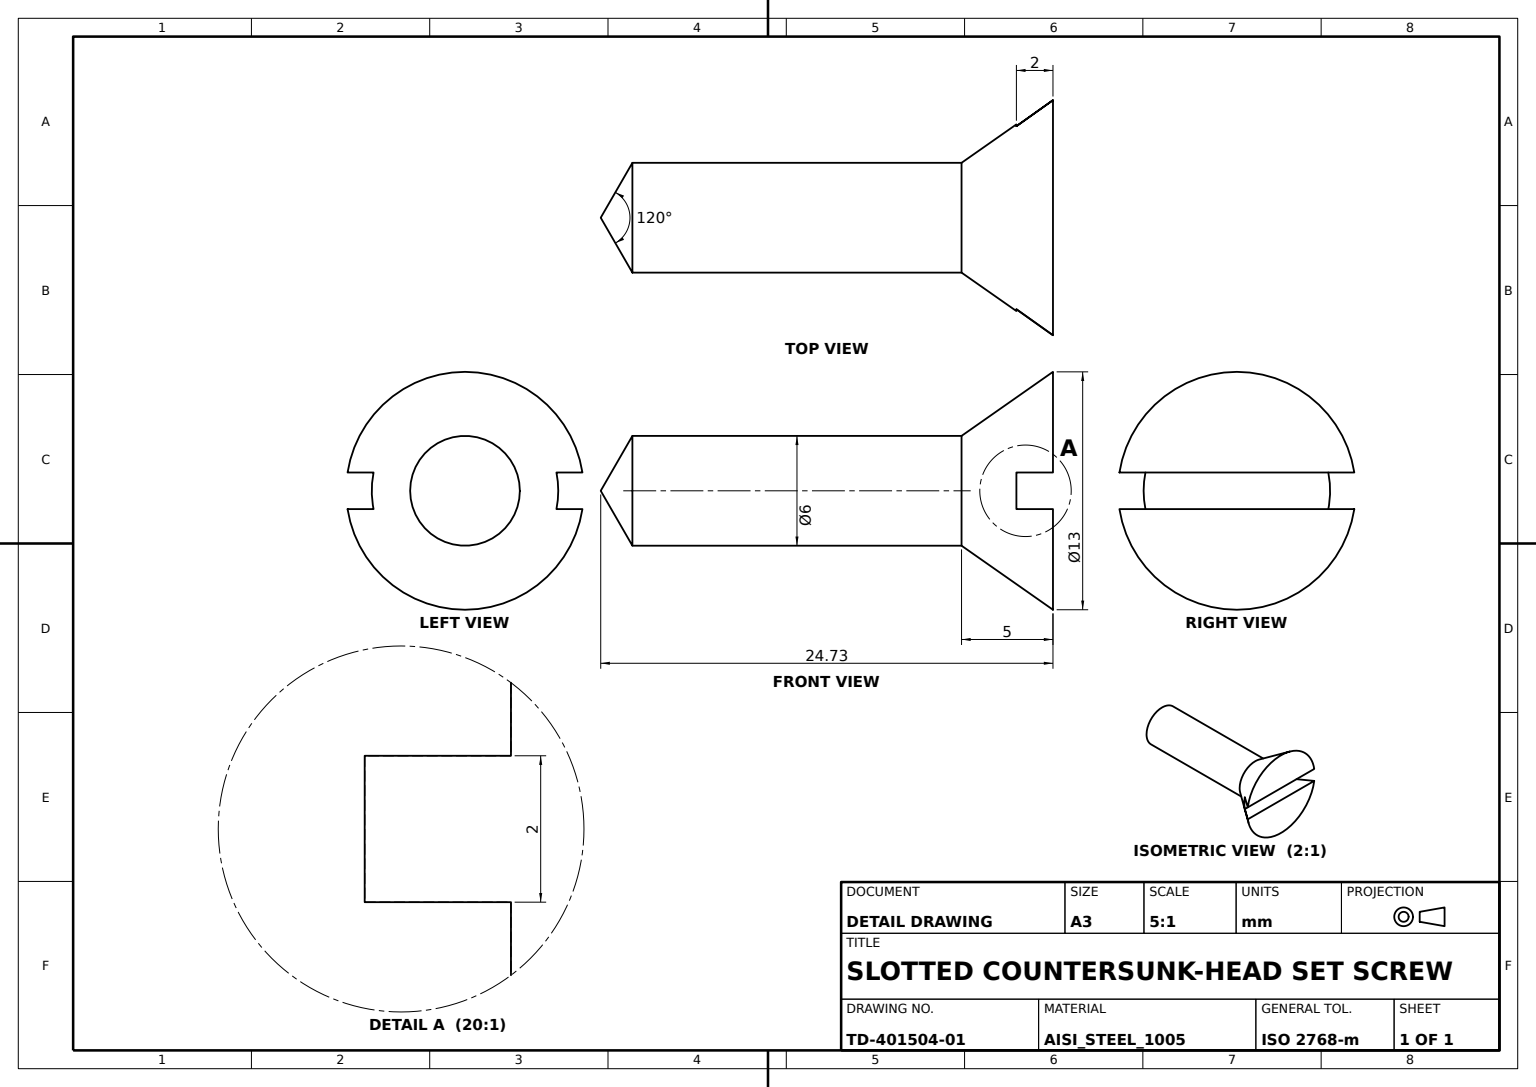
ISO-10303-21;
HEADER;
FILE_DESCRIPTION((''),'2;1');
FILE_NAME('','',(''),(''),'','','');
FILE_SCHEMA(('AUTOMOTIVE_DESIGN'));
ENDSEC;
DATA;
#1=APPLICATION_CONTEXT('');
#2=PRODUCT_CONTEXT('',#1,'mechanical');
#3=PRODUCT('','','',(#2));
#4=PRODUCT_DEFINITION_FORMATION('','',#3);
#5=PRODUCT_DEFINITION_CONTEXT('',#1,'design');
#6=PRODUCT_DEFINITION('','',#4,#5);
#7=PRODUCT_DEFINITION_SHAPE('','',#6);
#8=(LENGTH_UNIT()NAMED_UNIT(*)SI_UNIT(.MILLI.,.METRE.));
#9=(NAMED_UNIT(*)PLANE_ANGLE_UNIT()SI_UNIT($,.RADIAN.));
#10=(NAMED_UNIT(*)SI_UNIT($,.STERADIAN.)SOLID_ANGLE_UNIT());
#11=UNCERTAINTY_MEASURE_WITH_UNIT(LENGTH_MEASURE(0.005),#8,'distance_accuracy_value','');
#12=(GEOMETRIC_REPRESENTATION_CONTEXT(3)GLOBAL_UNCERTAINTY_ASSIGNED_CONTEXT((#11))GLOBAL_UNIT_ASSIGNED_CONTEXT((#8,#9,#10))REPRESENTATION_CONTEXT('',''));
#13=CARTESIAN_POINT('',(-13.646654,0.,-3.));
#14=VERTEX_POINT('',#13);
#15=CARTESIAN_POINT('',(-13.646654,0.,0.));
#16=DIRECTION('',(1.,0.,0.));
#17=DIRECTION('',(0.,0.,-1.));
#18=AXIS2_PLACEMENT_3D('',#15,#16,#17);
#19=CIRCLE('',#18,3.);
#20=EDGE_CURVE('',#14,#14,#19,.T.);
#21=ORIENTED_EDGE('',*,*,#20,.T.);
#22=EDGE_LOOP('',(#21));
#23=FACE_BOUND('',#22,.T.);
#24=CARTESIAN_POINT('',(4.353346,0.,-3.));
#25=VERTEX_POINT('',#24);
#26=CARTESIAN_POINT('',(4.353346,0.,0.));
#27=AXIS2_PLACEMENT_3D('',#26,#16,#17);
#28=CIRCLE('',#27,3.);
#29=EDGE_CURVE('',#25,#25,#28,.T.);
#30=ORIENTED_EDGE('',*,*,#29,.F.);
#31=EDGE_LOOP('',(#30));
#32=FACE_BOUND('',#31,.T.);
#33=CARTESIAN_POINT('',(0.,0.,0.));
#34=AXIS2_PLACEMENT_3D('',#33,#16,#17);
#35=CYLINDRICAL_SURFACE('',#34,3.);
#36=ADVANCED_FACE('',(#23,#32),#35,.T.);
#37=ORIENTED_EDGE('',*,*,#20,.F.);
#38=EDGE_LOOP('',(#37));
#39=FACE_BOUND('',#38,.T.);
#40=CARTESIAN_POINT('',(-16.646654,-1.,-5.001));
#41=VERTEX_POINT('',#40);
#42=CARTESIAN_POINT('',(-16.646654,1.,-5.001));
#43=VERTEX_POINT('',#42);
#44=CARTESIAN_POINT('',(-16.646654,0.,0.));
#45=DIRECTION('',(-1.,0.,0.));
#46=DIRECTION('',(0.,0.,1.));
#47=AXIS2_PLACEMENT_3D('',#44,#45,#46);
#48=CIRCLE('',#47,5.1);
#49=EDGE_CURVE('',#41,#43,#48,.F.);
#50=ORIENTED_EDGE('',*,*,#49,.T.);
#51=CARTESIAN_POINT('',(-18.646654,1.,-6.422616));
#52=VERTEX_POINT('',#51);
#53=CARTESIAN_POINT('',(-17.312348,1.,-5.47621));
#54=CARTESIAN_POINT('',(-17.979237,1.,-5.949795));
#55=B_SPLINE_CURVE_WITH_KNOTS('',3,(#42,#53,#54,#51),.UNSPECIFIED.,.F.,.F.,(4,4),(0.027715114,0.030169137),.UNSPECIFIED.);
#56=EDGE_CURVE('',#43,#52,#55,.T.);
#57=ORIENTED_EDGE('',*,*,#56,.T.);
#58=CARTESIAN_POINT('',(-18.646654,1.,6.422616));
#59=VERTEX_POINT('',#58);
#60=CARTESIAN_POINT('',(-18.646654,0.,0.));
#61=AXIS2_PLACEMENT_3D('',#60,#16,#17);
#62=CIRCLE('',#61,6.5);
#63=EDGE_CURVE('',#52,#59,#62,.T.);
#64=ORIENTED_EDGE('',*,*,#63,.T.);
#65=CARTESIAN_POINT('',(-16.646654,1.,5.001));
#66=VERTEX_POINT('',#65);
#67=CARTESIAN_POINT('',(-17.979241,1.,5.949798));
#68=CARTESIAN_POINT('',(-17.312364,1.,5.476222));
#69=B_SPLINE_CURVE_WITH_KNOTS('',3,(#58,#67,#68,#65),.UNSPECIFIED.,.F.,.F.,(4,4),(0.009653863,0.012107633),.UNSPECIFIED.);
#70=EDGE_CURVE('',#59,#66,#69,.T.);
#71=ORIENTED_EDGE('',*,*,#70,.T.);
#72=CARTESIAN_POINT('',(-16.646654,-1.,5.001));
#73=VERTEX_POINT('',#72);
#74=EDGE_CURVE('',#66,#73,#48,.F.);
#75=ORIENTED_EDGE('',*,*,#74,.T.);
#76=CARTESIAN_POINT('',(-18.646654,-1.,6.422616));
#77=VERTEX_POINT('',#76);
#78=CARTESIAN_POINT('',(-17.312348,-1.,5.47621));
#79=CARTESIAN_POINT('',(-17.979237,-1.,5.949795));
#80=B_SPLINE_CURVE_WITH_KNOTS('',3,(#72,#78,#79,#76),.UNSPECIFIED.,.F.,.F.,(4,4),(0.027715114,0.030169137),.UNSPECIFIED.);
#81=EDGE_CURVE('',#73,#77,#80,.T.);
#82=ORIENTED_EDGE('',*,*,#81,.T.);
#83=CARTESIAN_POINT('',(-18.646654,-1.,-6.422616));
#84=VERTEX_POINT('',#83);
#85=EDGE_CURVE('',#77,#84,#62,.T.);
#86=ORIENTED_EDGE('',*,*,#85,.T.);
#87=CARTESIAN_POINT('',(-17.979241,-1.,-5.949798));
#88=CARTESIAN_POINT('',(-17.312364,-1.,-5.476222));
#89=B_SPLINE_CURVE_WITH_KNOTS('',3,(#83,#87,#88,#40),.UNSPECIFIED.,.F.,.F.,(4,4),(0.009653863,0.012107633),.UNSPECIFIED.);
#90=EDGE_CURVE('',#84,#41,#89,.T.);
#91=ORIENTED_EDGE('',*,*,#90,.T.);
#92=EDGE_LOOP('',(#50,#57,#64,#71,#75,#82,#86,#91));
#93=FACE_BOUND('',#92,.T.);
#94=AXIS2_PLACEMENT_3D('',#15,#45,#46);
#95=CONICAL_SURFACE('',#94,3.,0.610725964);
#96=ADVANCED_FACE('',(#39,#93),#95,.T.);
#97=CARTESIAN_POINT('',(-16.646654,1.,7.));
#98=VECTOR('',#17,1000.);
#99=LINE('',#97,#98);
#100=EDGE_CURVE('',#43,#66,#99,.F.);
#101=ORIENTED_EDGE('',*,*,#100,.F.);
#102=ORIENTED_EDGE('',*,*,#49,.F.);
#103=CARTESIAN_POINT('',(-16.646654,-1.,7.));
#104=LINE('',#103,#98);
#105=EDGE_CURVE('',#41,#73,#104,.F.);
#106=ORIENTED_EDGE('',*,*,#105,.T.);
#107=ORIENTED_EDGE('',*,*,#74,.F.);
#108=EDGE_LOOP('',(#101,#102,#106,#107));
#109=FACE_BOUND('',#108,.T.);
#110=AXIS2_PLACEMENT_3D('',#103,#45,#46);
#111=PLANE('',#110);
#112=ADVANCED_FACE('',(#109),#111,.T.);
#113=ORIENTED_EDGE('',*,*,#85,.F.);
#114=CARTESIAN_POINT('',(-18.646654,-1.,7.));
#115=LINE('',#114,#98);
#116=EDGE_CURVE('',#77,#84,#115,.T.);
#117=ORIENTED_EDGE('',*,*,#116,.T.);
#118=EDGE_LOOP('',(#113,#117));
#119=FACE_BOUND('',#118,.T.);
#120=CARTESIAN_POINT('',(-18.646654,6.5,0.));
#121=AXIS2_PLACEMENT_3D('',#120,#45,#46);
#122=PLANE('',#121);
#123=ADVANCED_FACE('',(#119),#122,.T.);
#124=ORIENTED_EDGE('',*,*,#63,.F.);
#125=CARTESIAN_POINT('',(-18.646654,1.,7.));
#126=LINE('',#125,#98);
#127=EDGE_CURVE('',#59,#52,#126,.T.);
#128=ORIENTED_EDGE('',*,*,#127,.F.);
#129=EDGE_LOOP('',(#124,#128));
#130=FACE_BOUND('',#129,.T.);
#131=ADVANCED_FACE('',(#130),#122,.T.);
#132=CARTESIAN_POINT('',(6.085396,0.,0.));
#133=VERTEX_POINT('',#132);
#134=VERTEX_LOOP('',#133);
#135=FACE_BOUND('',#134,.T.);
#136=ORIENTED_EDGE('',*,*,#29,.T.);
#137=EDGE_LOOP('',(#136));
#138=FACE_BOUND('',#137,.T.);
#139=AXIS2_PLACEMENT_3D('',#132,#45,#46);
#140=CONICAL_SURFACE('',#139,0.,1.047197551);
#141=ADVANCED_FACE('',(#135,#138),#140,.T.);
#142=ORIENTED_EDGE('',*,*,#70,.F.);
#143=ORIENTED_EDGE('',*,*,#127,.T.);
#144=ORIENTED_EDGE('',*,*,#56,.F.);
#145=ORIENTED_EDGE('',*,*,#100,.T.);
#146=EDGE_LOOP('',(#142,#143,#144,#145));
#147=FACE_BOUND('',#146,.T.);
#148=DIRECTION('',(0.,-1.,0.));
#149=AXIS2_PLACEMENT_3D('',#97,#148,#17);
#150=PLANE('',#149);
#151=ADVANCED_FACE('',(#147),#150,.T.);
#152=ORIENTED_EDGE('',*,*,#81,.F.);
#153=ORIENTED_EDGE('',*,*,#105,.F.);
#154=ORIENTED_EDGE('',*,*,#90,.F.);
#155=ORIENTED_EDGE('',*,*,#116,.F.);
#156=EDGE_LOOP('',(#152,#153,#154,#155));
#157=FACE_BOUND('',#156,.T.);
#158=DIRECTION('',(0.,1.,0.));
#159=AXIS2_PLACEMENT_3D('',#114,#158,#46);
#160=PLANE('',#159);
#161=ADVANCED_FACE('',(#157),#160,.T.);
#162=CLOSED_SHELL('',(#36,#96,#112,#123,#131,#141,#151,#161));
#163=MANIFOLD_SOLID_BREP('',#162);
#164=ADVANCED_BREP_SHAPE_REPRESENTATION('',(#163),#12);
#165=SHAPE_DEFINITION_REPRESENTATION(#7,#164);
ENDSEC;
END-ISO-10303-21;
